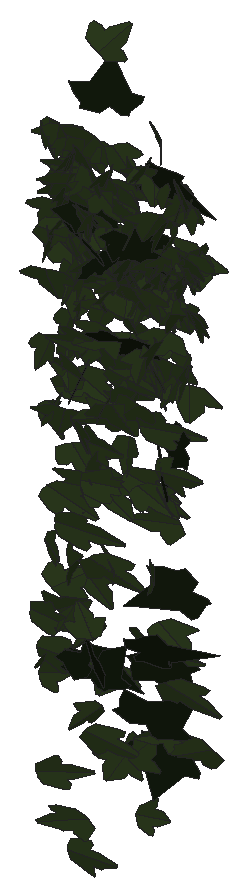
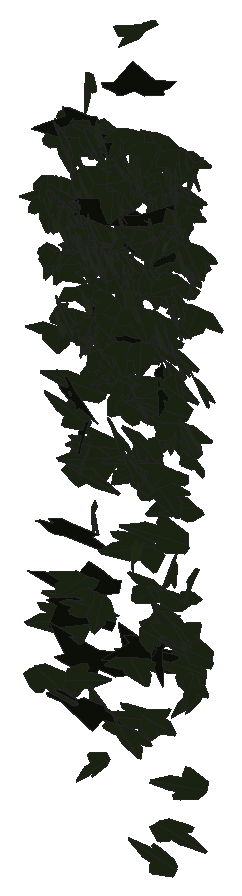
# SketchUp Ruby script. Lengths in millimetres.
U = 1.mm
M = Sketchup.active_model
def pt(a) = Geom::Point3d.new(a.map { |v| v * U })
def face(e, loops, mat)
  f = e.add_face(loops[0].map { |a| pt(a) })
  loops[1..].each { |l| e.add_face(l.map { |a| pt(a) }).erase! }
  f.material = f.back_material = mat if mat
  f
end
# faces: each face lists its corners as indices into pts; further lists are holes
def faces(e, pts, list, mat = nil) = list.each { |f| face(e, (f[0].is_a?(Array) ? f : [f]).map { |l| l.map { |i| pts[i] } }, mat) }
# xy, xz, yz: faces in a plane at the given z, y or x. An outline is a flat list of corners, or four numbers for a rectangle; further outlines are holes
def ring(l) = l.size == 4 ? [[l[0], l[1]], [l[2], l[1]], [l[2], l[3]], [l[0], l[3]]] : l.each_slice(2).to_a
def flat(e, list, mat, &to3) = list.each { |f| face(e, (f[0].is_a?(Array) ? f : [f]).map { |l| ring(l).map { |u, v| to3.(u, v) } }, mat) }
def xy(e, z, list, mat = nil) = flat(e, list, mat) { |x, y| [x, y, z] }
def xz(e, y, list, mat = nil) = flat(e, list, mat) { |x, z| [x, y, z] }
def yz(e, x, list, mat = nil) = flat(e, list, mat) { |y, z| [x, y, z] }
def lines(e, pts, list) = list.each { |a, b| e.add_line(pt(pts[a]), pt(pts[b])) }
# prism: a flat outline (further loops are holes) pulled along v
def prism(e, loops, v, mat = nil)
  f = face(e, loops, mat); d = Geom::Vector3d.new(v.map { |x| x * U })
  f.pushpull(f.normal.samedirection?(d) ? d.length : -d.length)
end
def box(e, o, s, mat = nil) = prism(e, [[o, [o[0] + s[0], o[1], o[2]], [o[0] + s[0], o[1] + s[1], o[2]], [o[0], o[1] + s[1], o[2]]]], [0, 0, s[2]], mat)
def at(x, y, z, deg = 0) = Geom::Transformation.translation(pt([x, y, z])) * Geom::Transformation.rotation(ORIGIN, Z_AXIS, deg.degrees)
def axes(o, x, y, z) = Geom::Transformation.new([*x, 0, *y, 0, *z, 0, *pt(o).to_a, 1])
def part(name) = M.definitions.add(name)
# library, detail: a bought-in or finely detailed component or shape, given as its bounding box
def library(name, o, s) = part(name).tap { |d| box(d.entities, o, s) }
def detail(e, o, s) = box(e.add_group.entities, o, s)
def put(e, d, t, mat = nil) = e.add_instance(d, t).tap { |i| i.material = mat if mat }
def group(e, t, mat = nil) = e.add_group.tap { |g| g.transformation = t; g.material = mat if mat }.entities
root = M.entities
M.materials.add("efeu1").color = [18, 25, 13]
M.materials.add("efeu2").color = [43, 57, 29]
c1 = part("ivyleaf_10")
p = [[0,12.8,-0.8],[-1.5,51.3,-10.9],[-4.9,51,-11.6],[-13.6,26.5,-7.3],[-13.2,15.9,-4.6],[-21.1,19.3,-7.2],
  [-29.5,16.3,-8.3],[-29.2,8.3,-6.2],[-19.7,-9.8,0.5],[-7.6,-13,4],[1,-12.2,5.8],[-0.4,51.1,-11.1],
  [-1.5,51.1,-10.9],[1,-12.4,5.9],[16.9,-12.4,3.5],[35.1,9.1,-5.1],[35,12.9,-6.1],[20.5,16.4,-4.9],
  [15.8,15,-3.8],[15.3,27.6,-7.1],[12.8,31.3,-7.8]]
faces(c1.entities,p,[[0,1,2,3,4,5,6,7,8,9,10],[11,12,0,13,14,15,16,17,18,19,20]],"efeu2")
c2 = part("ivyleaf_9")
p = [[39.1,54.8,31.7],[34.5,51.8,30.2],[-5.3,25.2,17.3],[-17.9,28.3,20.9],[-21.6,21.7,17],[-20.2,4.3,5.3],
  [-22.9,-0.3,2.5],[-17.1,-4,-0.6],[-2,-2.1,-1.2],[-0.7,-15.4,-10.1],[16.6,-22.3,-16.7],[21.1,-15.1,-12.5],
  [32.7,-10.7,-11],[46.1,-1.8,-6.6],[30.8,11.2,3.8]]
faces(c2.entities,p,[[0,1,2,3,4,5,6,7,8,9,10,11,12,13,14]],"efeu1")
put(root,c1,axes([1869.2,1029.3,798.4],[0.90738,-0.48267,0.05189],[0.05263,-0.04561,-0.67832],[0.92241,0.47741,-0.01234]))
put(root,c1,axes([1871.8,1032,897.3],[-1.24405,-0.13361,-0.11217],[0.20532,0.03226,-0.6671],[0.26092,-0.66243,-0.00987]))
put(root,c1,axes([1875.6,1030.7,519.9],[-0.37912,0.53611,0.3744],[-0.30349,0.33975,-0.57133],[-1.20694,-0.25383,0.02606]))
put(root,c1,axes([1874.4,1033.8,369],[-0.21212,-0.54646,-0.44472],[0.17012,0.43564,-0.55771],[1.33007,-0.14287,0.00041]))
put(root,c1,axes([1874.3,1024.3,1105.1],[-0.16268,0.70253,0.12456],[-0.12748,0.117,-0.70583],[-1.35191,-0.09557,0.05157]))
put(root,c1,axes([1879.6,1037.5,989.3],[1.27986,0.02095,-0.20491],[-0.38647,0.18461,-0.64756],[0.06565,0.67833,0.18256]))
put(root,c1,axes([1876.4,1025.5,342.8],[-0.0711,0.23931,0.73813],[-0.18187,0.73194,-0.24214],[-1.46555,-0.10244,-0.00576]))
put(root,c1,axes([1879.4,1022.1,952.3],[0.18952,-0.45863,-0.5924],[0.06095,0.59967,-0.45888],[1.42455,0.03536,0.09845]))
put(root,c1,axes([1861.4,1048.1,698.6],[0.73815,-0.23679,0.45324],[0.79308,-0.18337,-0.45238],[0.56409,0.56765,0.04293]))
put(root,c1,axes([1875.8,1027.5,702.7],[0.39878,-0.71333,0.09203],[0.04553,0.10271,0.74168],[-1.36811,-0.20451,0.05151]))
put(root,c1,axes([1857.3,1035.8,413.5],[0.02097,0.0114,0.70069],[1.31077,0.12931,-0.01293],[-0.24643,0.68875,-0.00917]))
put(root,c1,axes([1887.8,1035.7,973.4],[0.23825,-0.69334,0.05727],[0.03936,-0.05446,-0.70447],[1.32347,0.12643,0.01064]))
put(root,c1,axes([1900,1017.8,1106.3],[0.50659,-0.48712,-0.4683],[-0.4436,0.40624,-0.55505],[1.20709,0.35373,-0.00744]))
put(root,c1,axes([1890,1046,835.6],[0.77843,-0.48828,0.13906],[0.14957,-0.11552,-0.63681],[0.95459,0.41627,-0.01362]))
put(root,c1,axes([1897,1032,1032.3],[-0.51019,-0.65992,-0.06819],[0.04332,0.06435,-0.71228],[1.2619,-0.26902,-0.00312]))
put(root,c1,axes([1901.4,1025.6,716.5],[-1.11368,-0.33892,0.084],[-0.12948,-0.05012,-0.67616],[0.65181,-0.58903,0.00921]))
put(root,c1,axes([1893.6,1042.6,804.4],[0.2337,0.61212,-0.19031],[-0.1827,-0.17402,-0.62168],[-1.20623,0.14495,0.05729]))
put(root,c1,axes([1914.6,1035.5,145.8],[0.70854,0.0556,-0.56665],[-1.0806,-0.01434,-0.37444],[-0.08097,0.67785,0.03856]))
put(root,c1,axes([1900.4,1028.7,1110.1],[-0.96496,-0.51288,0.04323],[0.11399,-0.11907,-0.71008],[0.97292,-0.49474,0.12607]))
put(root,c1,axes([1899.9,1040.7,922.4],[0.81679,-0.52205,-0.12273],[-0.09683,0.11685,-0.67494],[1.01605,0.43081,0.03434]))
put(root,c1,axes([1883,1019.7,208],[-0.12187,-0.11847,0.71745],[0.66916,0.62539,0.13465],[-1.21141,0.35737,0.0022]))
put(root,c1,axes([1878.7,1024.3,966.6],[-0.35032,-0.14395,-0.67044],[1.20953,0.22489,-0.22277],[0.49012,-0.65787,0.07055]))
put(root,c1,axes([1902.7,1028.5,1030.1],[0.14499,-0.70911,-0.035],[0.02921,0.03684,-0.71293],[1.3509,0.07531,0.01917]))
put(root,c1,axes([1902.1,1042.7,812.7],[0.84625,-0.4996,-0.08924],[-0.08285,0.08067,-0.66848],[0.96233,0.44628,0.02093]))
put(root,c1,axes([1921.6,1019.6,778.5],[0.10379,-0.07883,-0.71109],[-0.96747,0.49756,-0.09414],[0.95815,0.51094,-0.01803]))
put(root,c1,axes([1902,1034.8,437.4],[0.87978,-0.51846,-0.03595],[-0.04796,0.0257,-0.69461],[0.98793,0.46294,-0.0017]))
put(root,c1,axes([1904.6,1038.2,892.7],[0.49545,-0.64141,-0.04392],[-0.02861,0.0413,-0.69222],[1.22326,0.26075,0.0016]))
put(root,c1,axes([1909.4,1024.3,1048.7],[-0.79443,-0.57764,0.05217],[-0.05687,-0.04278,-0.71267],[1.10237,-0.41849,0.00083]))
put(root,c1,axes([1911.8,1030.2,1057.9],[-1.34835,-0.08584,0.09967],[-0.18559,-0.0237,-0.71355],[0.16801,-0.71505,0.01169]))
put(root,c1,axes([1893,1037,432.7],[-1.03722,-0.17404,0.38096],[0.70107,0.09836,0.5719],[-0.37937,0.65762,0.01528]))
put(root,c1,axes([1887.5,1041.8,937.6],[0.87129,0.2454,0.46092],[0.75076,0.23911,-0.51911],[-0.65117,0.60404,0.01823]))
put(root,c1,axes([1923.8,1025.5,1002.4],[-0.81102,0.38818,0.4143],[-0.78257,0.14618,-0.55989],[-0.74506,-0.57608,0.1371]))
put(root,c1,axes([1914.5,1029.9,1004.8],[-1.23448,0.26015,0.1042],[-0.16954,0.05768,-0.69857],[-0.50569,-0.65441,-0.02015]))
put(root,c1,axes([1912.4,1022.8,1084.5],[0.37192,-0.65065,-0.2868],[-0.0069,0.29652,-0.67517],[1.35327,0.18033,0.07538]))
put(root,c1,axes([1918.7,1025.1,1092.9],[-0.98634,0.43433,0.25704],[-0.42293,0.13441,-0.67517],[-0.8624,-0.56266,0.03713]))
put(root,c1,axes([1893.6,1027.9,474.2],[0.72081,0.16976,-0.59681],[0.89097,0.38073,0.40538],[0.77507,-0.59554,0.08903]))
put(root,c1,axes([1913.9,1024.8,1080.8],[-0.01475,-0.69357,-0.19751],[0.05754,0.19703,-0.69308],[1.37127,-0.01573,0.02696]))
put(root,c1,axes([1883.2,1023.3,377.6],[-0.02616,0.02185,-0.77796],[1.4554,-0.14422,-0.01756],[-0.27527,-0.7646,-0.01892]))
put(root,c1,axes([1907.8,1044.4,879.5],[1.24386,-0.13508,0.0773],[0.13939,-0.0275,-0.66727],[0.26135,0.65754,-0.01202]))
put(root,c1,axes([1920.8,1030.1,912.8],[0.60241,-0.53759,-0.39212],[-0.23928,0.37809,-0.61983],[1.24358,0.33316,0.07069]))
put(root,c1,axes([1913.7,1050.7,867.1],[0.24232,-0.63004,0.19354],[0.19168,-0.1762,-0.63986],[1.23966,0.1504,0.0611]))
put(root,c1,axes([1911.6,1033.9,959.6],[-0.23603,0.68197,0.07052],[0.00464,0.0721,-0.69298],[-1.30483,-0.12311,-0.01522]))
put(root,c1,axes([1897.8,1035.7,746.9],[-0.30774,-0.16716,0.65401],[0.79369,0.50409,0.23194],[-1.01024,0.44696,-0.017]))
put(root,c1,axes([1917.7,1017.1,514.2],[0.15685,-0.2596,-0.77329],[0.08281,0.77752,-0.25638],[1.55023,-0.01526,0.09194]))
put(root,c1,axes([1922.6,1027.9,977.8],[0.15997,0.2002,-0.74136],[-0.17654,0.74297,0.19012],[1.45079,0.06834,0.10488]))
put(root,c1,axes([1937.5,1023.1,825.4],[0.52602,0.02308,-0.64568],[-1.17735,0.21208,-0.25722],[0.35478,0.66956,0.10373]))
put(root,c1,axes([1910.1,1027.2,1049.3],[-1.13091,-0.32991,-0.26224],[0.57378,-0.01601,-0.66299],[0.56046,-0.64931,0.14959]))
put(root,c1,axes([1932.3,1032.3,627.5],[-1.07139,-0.21896,0.34265],[-0.58476,-0.15427,-0.60337],[0.50694,-0.64071,0.02818]))
put(root,c1,axes([1897.3,1018.7,605.3],[0.64467,0.28691,0.5898],[0.86938,0.37315,-0.44386],[-0.89575,0.56865,-0.00632]))
put(root,c1,axes([1925.6,1033.7,973.2],[-0.89693,-0.50798,0.10975],[-0.02806,-0.13503,-0.68828],[0.98869,-0.46466,0.08003]))
put(root,c1,axes([1916.8,1028.6,706.1],[-0.77464,0.51378,-0.15067],[0.16318,-0.12427,-0.65539],[-1.00585,-0.41584,0.00971]))
put(root,c1,axes([1919,1025.3,1063],[1.26036,-0.30568,0.00153],[0.01934,0.01837,-0.72908],[0.58145,0.66198,0.02094]))
put(root,c2,axes([1932.9,1014.6,774.3],[-0.24355,0.15475,-0.77354],[-1.03911,0.54826,0.2],[1.08368,0.56049,0.01793]))
put(root,c1,axes([1909.5,1039.3,659],[1.01715,0.34047,0.27122],[0.42607,0.15334,-0.63363],[-0.7105,0.57938,0.00831]))
put(root,c1,axes([1919.6,1037.7,989.8],[0.03741,-0.59176,-0.37503],[0.34064,0.36697,-0.56966],[1.28912,-0.0798,0.16141]))
put(root,c1,axes([1922.7,1035.2,964.5],[-1.30315,-0.08826,-0.11103],[0.2088,0.01732,-0.69037],[0.17107,-0.69344,-0.00311]))
put(root,c1,axes([1930.1,1047.7,299.9],[-0.16769,-0.42013,0.50884],[-0.11506,-0.50606,-0.4283],[1.25058,-0.1029,0.02882]))
put(root,c1,axes([1918.7,1022.7,1038.4],[-1.07164,-0.26725,-0.35085],[0.58386,0.17146,-0.62295],[0.60307,-0.6409,-0.02035]))
put(root,c2,axes([1904.6,1035.1,978.8],[0.71859,-0.64527,0.24174],[0.23485,-0.20787,-0.74761],[1.29022,0.39722,0.00145]))
put(root,c1,axes([1933.7,1043.5,928.2],[-0.33889,-0.66496,0.00959],[0.01809,-0.01247,-0.68827],[1.26555,-0.17789,0.01241]))
put(root,c1,axes([1955.1,1032.3,991.7],[0.51592,-0.01403,-0.65537],[-1.19211,0.20358,-0.26344],[0.36788,0.67937,0.06541]))
put(root,c2,axes([1946.9,1032.4,997.9],[-1.2663,-0.37347,0.21608],[0.40405,0.06237,0.76151],[-0.71491,0.69677,0.04765]))
put(root,c1,axes([1939.3,1042.1,420.2],[-0.05524,-0.42579,0.51823],[-0.0381,-0.51794,-0.42667],[1.27595,-0.0339,0.0097]))
put(root,c1,axes([1908.4,1027.1,557.9],[0.03304,-0.04195,0.81892],[1.4007,0.36199,0.00294],[-0.68817,0.73478,0.0453]))
put(root,c1,axes([1940.5,1023.1,426],[0.43203,0.6509,0.02879],[-0.01824,-0.02714,0.68935],[1.23987,-0.22721,0.00011]))
put(root,c1,axes([1913.6,1039.7,97.5],[0.22404,-0.05782,-0.69253],[1.16936,-0.31951,0.13112],[-0.61795,-0.62559,-0.00296]))
put(root,c1,axes([1937.7,1025.6,1065.2],[1.05261,-0.42964,-0.20857],[0.02297,0.33159,-0.65106],[0.90865,0.48933,0.25806]))
put(root,c1,axes([1945,1019.4,1115.2],[1.23119,-0.19465,-0.31456],[-0.4179,0.30792,-0.6421],[0.56658,0.65009,0.20995]))
put(root,c1,axes([1938.4,1026.4,1103.8],[-1.23328,-0.29707,-0.16107],[0.33988,-0.00533,-0.70864],[0.54599,-0.6677,0.07732]))
put(root,c1,axes([1920,1044.8,487.7],[1.09364,0.06195,0.46136],[0.86422,0.08666,-0.57722],[-0.19492,0.73181,0.02929]))
put(root,c2,axes([1955,1016.1,398.3],[0.444,0.0027,-0.75716],[-1.39505,0.19936,-0.22514],[0.36113,0.76679,0.0612]))
put(root,c1,axes([1946.9,1022.6,652.1],[-0.17277,0.27104,0.60208],[-0.40048,0.56418,-0.28571],[-1.19112,-0.229,0.00873]))
put(root,c1,axes([1942.1,1027.4,1003.2],[0.12581,-0.70793,-0.03914],[0.20415,0.04884,-0.70226],[1.33385,0.0593,0.11118]))
put(root,c1,axes([1924.9,1031.1,772.1],[0.7651,0.41206,0.50055],[0.69141,0.34465,-0.57549],[-1.02201,0.54164,-0.01461]))
put(root,c1,axes([1952.4,1045.3,872.3],[-1.01897,-0.36098,0.13926],[-0.14907,-0.13172,-0.64255],[0.72112,-0.5373,0.06395]))
put(root,c1,axes([1963.1,1037.1,918.4],[0.85012,0.24064,-0.45675],[-0.97884,0.15486,-0.42138],[-0.08551,0.61981,0.28262]))
put(root,c1,axes([1970.6,1035.5,731.3],[-0.56478,-0.17989,0.61317],[-0.92096,-0.37828,-0.34517],[0.79429,-0.56652,0.03577]))
put(root,c1,axes([1951.6,1039.9,820.8],[-0.44554,-0.60072,-0.16652],[0.14091,0.14982,-0.64457],[1.17801,-0.24513,0.01412]))
put(root,c1,axes([1965.2,1022.6,848.5],[1.04645,-0.14115,-0.43031],[-0.77415,0.14363,-0.56686],[0.37891,0.68327,0.03027]))
put(root,c1,axes([1935.1,1040.4,676.5],[-0.50971,0.06887,0.65345],[1.20446,-0.16273,0.27653],[0.3363,0.6872,0]))
put(root,c2,axes([1935.3,1023.7,389.8],[0.03833,-0.20481,-0.73651],[0.68448,0.65268,-0.17166],[1.28385,-0.34186,0.11351]))
put(root,c1,axes([1959.3,1038.2,751.4],[0.45401,-0.67456,0.04375],[0.03265,-0.04034,-0.71549],[1.2861,0.23915,0.00272]))
put(root,c2,axes([1948.8,1022,365.4],[-0.8567,0.16075,0.59626],[1.04883,-0.22842,0.47762],[0.53041,0.71132,0.01862]))
put(root,c1,axes([1941.4,1045.8,634.2],[0.50849,-0.29727,-0.61621],[0.75646,-0.471,0.39955],[-1.05982,-0.47881,-0.01046]))
put(root,c1,axes([1963.9,1042.1,898.5],[-0.07625,-0.66463,-0.04561],[0.01867,0.0451,-0.6658],[1.26776,-0.04064,0.00706]))
put(root,c1,axes([1962.7,1042.5,369.6],[1.11396,0.32787,-0.18661],[-0.325,-0.07689,-0.6707],[-0.64022,0.60951,0.01577]))
put(root,c2,axes([1964.5,1010,945.4],[-0.69895,0.64319,-0.28504],[-0.2727,0.24642,0.74065],[1.31088,0.39421,0.0021]))
put(root,c1,axes([1945.9,1037.8,979.3],[0.61143,0.31857,0.53996],[0.65471,0.41766,-0.45109],[-0.99751,0.4694,0.03491]))
put(root,c1,axes([1965.2,1033.5,987.2],[-0.28251,0.67141,-0.15233],[-0.09529,-0.16594,-0.68263],[-1.30684,-0.13305,0.08271]))
put(root,c1,axes([1971.9,1023,1079.4],[-0.10492,-0.67514,-0.28163],[0.00385,0.28228,-0.67711],[1.39223,-0.05166,-0.01935]))
put(root,c1,axes([1972.5,1039.1,813.2],[-1.09428,-0.34902,-0.06739],[0.10707,0.03718,-0.6726],[0.66799,-0.57771,-0.00258]))
put(root,c1,axes([1960.1,1043.2,518],[-0.39992,0.10814,0.66432],[0.80799,-0.51874,0.21873],[0.99401,0.46517,0.08948]))
put(root,c1,axes([1976.3,1044,932.3],[-0.71874,-0.57098,0.05906],[0.04805,-0.08715,-0.6811],[1.09144,-0.37217,0.06888]))
put(root,c2,axes([1975.9,1021.3,1177.3],[-1.13627,-0.25849,0.507],[0.89507,0.18966,0.65051],[-0.60987,0.75995,0.0101]))
put(root,c1,axes([1966.4,1025.8,1038.1],[0.82026,0.45239,0.33799],[0.08856,0.39528,-0.58841],[-1.07109,0.37913,0.21019]))
put(root,c1,axes([1981.4,1027.2,820.9],[-1.23012,-0.13021,0.09156],[-0.17089,-0.01792,-0.65933],[0.25014,-0.65255,-0.00016]))
put(root,c1,axes([1976.7,1043.7,913.1],[-0.59365,-0.60076,-0.06235],[0.12042,0.03728,-0.6758],[1.14319,-0.3159,0.03881]))
put(root,c1,axes([1979.5,1032,929.3],[-0.5486,0.57807,0.22661],[-0.23821,0.19062,-0.64545],[-1.15745,-0.31322,0.02543]))
put(root,c1,axes([1954.5,1025.2,281.7],[-0.5241,-0.01575,-0.69148],[1.31617,-0.01937,-0.27497],[-0.02316,-0.74405,0.0218]))
put(root,c1,axes([1958.9,1013.1,641.9],[0.09116,0.03506,0.74705],[0.83284,0.60574,-0.05648],[-1.15426,0.43983,0.01824]))
put(root,c1,axes([2002.4,1024.3,1038.4],[0.34132,0.00919,0.70771],[-1.32016,0.1474,0.17386],[-0.26775,-0.71505,0.04493]))
put(root,c1,axes([1971.8,1014.3,1260.1],[0.62985,0.25071,-0.71224],[0.56946,0.67044,0.37503],[1.31942,-0.40904,0.17814]))
put(root,c1,axes([1961.5,1022.7,527],[-0.94004,-0.07334,-0.62422],[1.18806,0.03515,-0.49807],[0.13921,-0.79522,0.03556]))
put(root,c1,axes([1984.3,1032.4,947.6],[-0.67759,0.5905,0.14518],[-0.19554,0.1074,-0.68879],[-1.14067,-0.36919,0.03183]))
put(root,c1,axes([1965.7,1018.6,634.7],[0.83196,0.41463,0.44634],[0.64025,0.29372,-0.60232],[-0.96665,0.5514,-0.01479]))
put(root,c1,axes([1985.6,1039.6,942.9],[0.76677,-0.5514,-0.11074],[-0.03267,0.1241,-0.68038],[1.06988,0.39897,0.05859]))
put(root,c1,axes([1987.6,1027.8,1054.6],[-1.12329,0.40233,-0.00681],[-0.13021,-0.11225,-0.70213],[-0.75467,-0.57948,0.13128]))
put(root,c1,axes([1986.6,1031.5,258.6],[1.27446,-0.14152,-0.14354],[-0.26775,0.02853,-0.68443],[0.27475,0.68426,-0.00115]))
put(root,c1,axes([1981.1,1027.4,747.1],[-1.20834,-0.34234,-0.28304],[0.47236,0.13607,-0.72131],[0.70111,-0.68169,-0.00184]))
put(root,c1,axes([1979.4,1039.6,923],[1.29431,-0.01999,0.0766],[0.15058,0.14965,-0.66341],[0.00501,0.66781,0.15096]))
put(root,c1,axes([2005.9,1026,1086.4],[-0.39237,0.11741,0.68981],[-1.08644,0.38766,-0.23659],[-0.77016,-0.60668,-0.01768]))
put(root,c1,axes([1982.3,1028.5,1061],[-1.29777,0.00203,-0.23138],[0.43876,-0.05572,-0.6799],[-0.03773,-0.71792,0.05211]))
put(root,c2,axes([1993.3,1020,853],[0.98689,0.41964,-0.39361],[-0.60776,-0.23085,-0.66682],[-0.91085,0.60871,0.01846]))
put(root,c1,axes([1981.9,1025.8,1110.1],[-0.81771,-0.53371,-0.25998],[0.58635,0.07387,-0.6608],[0.96579,-0.49672,0.18107]))
put(root,c1,axes([1993.5,1041.3,939.8],[0.17215,-0.68841,-0.00253],[-0.02961,0.00051,-0.69416],[1.30986,0.09049,-0.01536]))
put(root,c1,axes([1982,1047.5,690.6],[0.92764,-0.40839,0.33505],[0.46982,-0.22695,-0.63574],[0.88881,0.54619,-0.01364]))
put(root,c1,axes([1992.6,1042.3,941.2],[-1.11505,-0.32862,-0.12945],[0.27672,0.00409,-0.66847],[0.61261,-0.6,0.06634]))
put(root,c1,axes([1999.8,1029.5,1007],[0.42642,-0.5516,-0.38764],[-0.22824,0.36937,-0.59491],[1.26265,0.25305,0.02338]))
put(root,c1,axes([2009.6,1028.6,760.7],[-1.16475,-0.05726,0.34253],[-0.64583,-0.04897,-0.61449],[0.14053,-0.69962,0.01498]))
put(root,c1,axes([2000.2,1027,961.1],[0.10598,-0.70385,0.02087],[-0.0027,-0.02105,-0.70604],[1.34015,0.05562,-0.00307]))
put(root,c1,axes([1992.6,1032.3,890],[1.26355,0.24782,-0.06113],[0.10675,0.02453,0.70865],[0.47392,-0.66627,0.00335]))
put(root,c1,axes([2005.4,1035.2,1023.3],[-1.26552,0.20978,0.13214],[-0.25343,0.01687,-0.69686],[-0.39803,-0.67774,0.02356]))
put(root,c1,axes([2001.4,1044.2,940.4],[0.39991,-0.64611,0.10223],[0.02853,-0.10259,-0.6792],[1.24464,0.20995,-0.01727]))
put(root,c1,axes([1992.3,1032.7,780.8],[-0.50678,-0.36141,-0.54956],[0.6369,0.43598,-0.44886],[1.0777,-0.4276,0.00684]))
put(root,c1,axes([2006.1,1032.6,941.7],[-0.50964,0.46878,0.42568],[-0.38882,0.3735,-0.53984],[-1.14068,-0.33676,-0.00617]))
put(root,c1,axes([2006.4,1032.8,909.7],[0.58348,-0.61002,-0.07226],[-0.07599,0.0608,-0.68268],[1.16664,0.30905,-0.00833]))
put(root,c1,axes([2010.3,1043.9,790.8],[-0.62956,-0.59425,0.12127],[-0.08388,-0.11421,-0.67991],[1.15124,-0.33329,0.01678]))
put(root,c1,axes([1994.4,1039,843.2],[1.24631,0.18999,0.14129],[0.26014,0.03595,-0.68184],[-0.36794,0.66895,-0.00349]))
put(root,c1,axes([1984.8,1031.4,796.9],[-0.50888,-0.01656,-0.65176],[1.23311,-0.08527,-0.26363],[-0.13831,-0.6993,0.04759]))
put(root,c1,axes([2012.6,1037.9,941.4],[-0.33098,-0.6615,0.03756],[0.02853,-0.04275,-0.6835],[1.26066,-0.17271,0.02533]))
put(root,c1,axes([2005.4,1036.6,868.8],[-1.03339,0.35357,-0.15906],[0.23506,-0.10172,-0.64772],[-0.69943,-0.55658,0.01734]))
put(root,c1,axes([2010.5,1044,921.5],[0.56074,-0.61908,-0.05153],[0.02009,-0.05203,0.6855],[-1.18214,-0.29454,-0.01279]))
put(root,c1,axes([2023.2,1036.5,432.2],[-1.24818,0.39283,0.12554],[-0.20916,0.06083,-0.76447],[-0.75651,-0.66496,0.00423]))
put(root,c1,axes([2018.3,1034.7,911],[0.82907,-0.50722,0.1045],[0.1208,-0.08323,-0.66858],[0.97818,0.44018,-0.006]))
put(root,c1,axes([2031.7,1036.2,816.2],[0.82737,-0.32539,-0.48302],[-0.58096,0.38602,-0.53477],[0.94397,0.52277,0.09424]))
put(root,c1,axes([2021.2,1032.2,834.4],[-0.33941,-0.63529,0.24202],[0.23343,-0.27617,-0.63455],[1.27262,-0.11878,0.18094]))
put(root,c1,axes([2025.3,1047.4,938.7],[0.21862,-0.66534,0.07138],[-0.00579,-0.07295,-0.67501],[1.27353,0.11389,-0.01532]))
put(root,c1,axes([2008,1033.7,269.9],[1.09189,-0.41831,-0.27874],[0.46401,-0.13834,0.7094],[-0.83663,-0.62266,0.02966]))
put(root,c1,axes([2030.5,1041.8,941.3],[1.17711,-0.11408,-0.25369],[-0.44229,0.12799,-0.62411],[0.29094,0.65613,0.07764]))
put(root,c1,axes([2028.4,1024.8,1103.6],[0.10808,-0.72834,-0.05716],[0.01238,0.05783,-0.73047],[1.39038,0.0561,0.01095]))
put(root,c2,axes([2007.1,1026.8,998.2],[-0.18019,-0.33999,-0.74396],[0.56861,0.68281,-0.35007],[1.4492,-0.31018,0.04485]))
put(root,c1,axes([2020.2,1022.8,925.3],[-1.2345,0.03739,-0.22953],[0.43738,-0.00107,-0.64962],[-0.06777,-0.68806,-0.01146]))
put(root,c1,axes([2027.3,1047.9,933.1],[0.72091,0.52939,-0.18848],[-0.23355,-0.14389,-0.65077],[-1.04367,0.39787,0.01543]))
put(root,c1,axes([2038.4,1030.7,822.2],[-0.7005,0.50743,0.34833],[-0.436,0.26376,-0.62629],[-1.08723,-0.43271,0.02672]))
put(root,c1,axes([2028.5,1024.9,195.2],[-0.04994,0.29922,0.63077],[-0.03315,0.63073,-0.29993],[-1.32828,-0.02699,-0.01623]))
put(root,c1,axes([2030.7,1039.5,972.9],[0.71409,-0.58849,0.03217],[0.11149,-0.00071,-0.69621],[1.11614,0.37658,0.04896]))
put(root,c1,axes([2037.1,1035.2,965.1],[-1.30479,0.0927,0.02838],[-0.06824,-0.05418,-0.68934],[-0.17143,-0.68402,0.05844]))
put(root,c1,axes([2041.9,1030.5,1035.2],[-0.72491,-0.58178,0.17553],[-0.13555,-0.163,-0.69478],[1.14857,-0.38642,0.02879]))
put(root,c1,axes([2010.1,1032,657.8],[0.45349,0.13975,0.65069],[1.1012,0.298,-0.27588],[-0.62586,0.62559,-0.01394]))
put(root,c1,axes([2030.2,1043.1,837.6],[0.14922,0.66805,0.02246],[0.0087,0.02208,-0.67263],[-1.27213,0.07851,-0.00197]))
put(root,c1,axes([2056.6,1037.4,610.2],[0.52707,-0.06751,-0.63438],[-1.1966,0.08832,-0.28387],[0.20577,0.68653,-0.02586]))
put(root,c1,axes([2039.7,1037,969.2],[-0.63311,-0.61988,-0.05908],[0.06719,0.0481,-0.70345],[1.18319,-0.33442,0.00833]))
put(root,c1,axes([2043.9,1026.7,1099.7],[-1.19282,-0.36102,0.03365],[-0.05459,-0.01763,-0.72329],[0.68792,-0.6274,0.00096]))
put(root,c1,axes([2040.7,1046,948],[0.18417,-0.62053,0.2652],[0.05908,-0.26354,-0.62796],[1.28297,0.10121,-0.00915]))
put(root,c1,axes([2045.7,1035.1,648.7],[-0.70762,0.5281,0.30284],[-0.34392,0.24311,-0.64581],[-1.10638,-0.41333,0.00707]))
put(root,c1,axes([2049.3,1027,1089.4],[0.95716,-0.56422,-0.30564],[-0.41439,0.21525,-0.75562],[1.14881,0.54774,-0.0179]))
put(root,c1,axes([2021.9,1037.6,640],[-0.71814,-0.02111,-0.58524],[1.11366,0.01436,-0.37779],[0.04474,-0.69619,0.00996]))
put(root,c1,axes([2044.9,1028.5,859.7],[0.14449,-0.70488,0.09799],[0.03861,-0.09636,-0.70889],[1.35388,0.07798,0.00976]))
put(root,c1,axes([2033.2,1040.8,959.9],[-0.93419,0.27056,-0.40221],[0.51,-0.32555,-0.54601],[-0.76878,-0.54473,0.12654]))
put(root,c1,axes([2050.5,1011.1,539.8],[0.00001,-0.08958,-0.67894],[-0.19439,0.67135,-0.08858],[1.28879,0.10126,-0.01336]))
put(root,c1,axes([2056.8,1044.2,313.6],[0.09857,0.09369,-0.70529],[-0.87743,-0.5342,-0.10482],[-1.03137,0.46342,0.02177]))
put(root,c1,axes([2050.7,1035.7,868.9],[0.8573,0.37582,-0.33486],[-0.59907,-0.14034,-0.58094],[-0.74757,0.54345,0.08154]))
put(root,c1,axes([2043.4,1027.2,806.5],[-0.49131,0.63815,0.07496],[-0.0555,0.06906,-0.68838],[-1.22161,-0.25979,0.00113]))
put(root,c2,axes([2052.5,1037.5,654.7],[-0.03045,-0.41579,0.66314],[0.2541,0.6521,0.41209],[-1.46782,0.12151,0.05758]))
put(root,c1,axes([2030,1026.2,647.9],[0.66816,0.35443,0.47626],[0.59941,0.35783,-0.49845],[-0.95776,0.4712,0.02029]))
put(root,c1,axes([2041.8,1025.9,1097],[1.16113,0.38909,-0.0028],[-0.01496,0.00711,-0.72353],[-0.74038,0.61006,0.01022]))
put(root,c1,axes([2051.1,1043.7,943.2],[0.65645,-0.55655,-0.19979],[-0.13958,0.18925,-0.65379],[1.11672,0.35081,0.03573]))
put(root,c2,axes([2050.3,1044.3,284.9],[-1.36287,-0.28278,-0.3521],[0.62764,0.1235,-0.76988],[0.58717,-0.78836,0.00569]))
put(root,c1,axes([2031.5,1043,910.8],[0.43062,-0.32432,0.5422],[1.00698,-0.21748,-0.35088],[0.65715,0.54578,0.18237]))
put(root,c1,axes([2052.6,1029.1,1027.8],[0.29207,-0.69055,0.08481],[0.06601,-0.07915,-0.7072],[1.32249,0.15646,0.01657]))
put(root,c1,axes([2042.4,1031.5,925.2],[-1.12804,-0.09398,-0.31926],[0.63316,-0.18537,-0.56305],[-0.01754,-0.6472,0.20763]))
put(root,c1,axes([2062,1038.2,829.1],[-1.2423,-0.09316,0.14039],[-0.25063,-0.06832,-0.65761],[0.20004,-0.66416,0.04796]))
put(root,c2,axes([2035.8,1023,329],[-0.67939,0.12119,0.75407],[1.35749,-0.24468,0.37698],[0.51967,0.79761,0.00107]))
put(root,c2,axes([2079.1,1035.4,725.3],[-0.43127,0.0833,-0.7197],[-1.34614,0.1379,0.23866],[0.29867,0.74182,0.03645]))
put(root,c1,axes([2059.1,1040,978.9],[-0.48474,-0.64705,0.0378],[0.02238,-0.04522,-0.69483],[1.23336,-0.25349,0.02747]))
put(root,c1,axes([2057.7,1014.5,1157.8],[0.59402,-0.4556,-0.5088],[-0.03513,0.55359,-0.50702],[1.29935,0.22325,0.2189]))
put(root,c1,axes([2056.5,1041.2,964],[0.39479,-0.65308,0.08528],[0.07619,-0.07674,-0.68508],[1.25119,0.21074,0.01481]))
put(root,c1,axes([2032.5,1035.9,734.1],[-0.26116,-0.08647,0.76358],[1.23158,0.40535,0.16219],[-0.78882,0.6615,0.00042]))
put(root,c2,axes([2045.2,1033,415.1],[-0.4162,-0.36976,-0.64994],[0.62624,0.56049,-0.42959],[1.27794,-0.39509,-0.00116]))
put(root,c1,axes([2038.2,1034.3,420.9],[-0.12236,-0.11668,0.69634],[1.1037,0.39011,0.11892],[-0.76648,0.58037,0.06007]))
put(root,c2,axes([2085.2,1040.9,522.9],[-1.47744,-0.06747,0.23343],[-0.43935,-0.03911,-0.77901],[0.14433,-0.80968,0.01818]))
put(root,c1,axes([2049.5,1039.4,457.2],[0.70957,0.50135,0.35477],[0.41004,0.28188,-0.62477],[-1.09462,0.43059,-0.00406]))
put(root,c2,axes([2034.5,1015.9,431.5],[0.55363,0.02408,0.75124],[1.41895,0.0929,-0.29167],[-0.18139,0.80022,0.01125]))
put(root,c1,axes([2064.5,1032.1,809.4],[0.73804,-0.55151,0.00364],[0.00437,-0.00284,-0.6742],[1.04965,0.3878,0.00025]))
put(root,c1,axes([2082.1,1046.9,896.3],[-1.0449,0.02235,-0.40135],[-0.76292,0.02003,0.54947],[0.05684,0.67978,-0.00299]))
put(root,c1,axes([2069.4,1028,1021.4],[0.24862,-0.67134,-0.19616],[-0.05897,0.1938,-0.68391],[1.32982,0.13411,0.00635]))
put(root,c2,axes([2037.7,1024.5,1098.5],[0.0477,-0.00634,-0.81179],[1.28552,0.4507,0.01734],[0.85709,-0.67564,0.01918]))
put(root,c1,axes([2075,1030.9,983],[-1.02157,0.44477,0.03747],[-0.18236,-0.05758,-0.68909],[-0.82968,-0.53498,0.10532]))
put(root,c1,axes([2072.4,1047.1,841.2],[0.77238,-0.54322,0.02309],[0.0233,-0.01968,-0.67808],[1.03453,0.40601,-0.00197]))
put(root,c1,axes([2081.9,1028.2,1071],[-1.30377,0.16311,0.18269],[-0.36737,-0.02557,-0.70096],[-0.28688,-0.70852,0.06735]))
put(root,c1,axes([2072.8,1039.6,980.7],[0.73123,-0.57202,-0.11484],[0.03907,0.15067,-0.68183],[1.1097,0.37162,0.09968]))
put(root,c1,axes([2077.9,1039.8,975.4],[1.03915,-0.39262,-0.12601],[-0.20955,0.06268,-0.67238],[0.75628,0.55684,-0.01316]))
put(root,c1,axes([2073,1039.9,909.8],[-0.48269,-0.58125,-0.24503],[0.33022,0.18962,-0.62941],[1.1542,-0.29733,0.07761]))
put(root,c1,axes([2096.7,1041.6,996.8],[-0.94171,0.16819,0.44755],[-0.90761,-0.21967,-0.44469],[0.06505,-0.62998,0.27454]))
put(root,c1,axes([2074.8,1023.7,916.3],[-0.11778,-0.32946,-0.66162],[0.33762,0.63791,-0.33424],[1.36556,-0.18613,0.02557]))
put(root,c1,axes([2079.4,1028.1,1072.1],[0.50774,-0.66212,-0.10822],[0.09055,0.13484,-0.7077],[1.27365,0.25437,0.09346]))
put(root,c1,axes([2081,1037.7,977.2],[-0.89727,0.51453,0.03959],[-0.06821,0.02085,-0.69775],[-0.97977,-0.47266,0.01232]))
put(root,c1,axes([2056,1033.7,682.7],[0.36622,-0.08872,-0.67192],[1.11198,-0.33226,0.21119],[-0.6537,-0.6149,-0.01717]))
put(root,c1,axes([2104.2,1046.3,304.2],[-0.89631,-0.11357,0.54585],[-0.96616,-0.20807,-0.48128],[0.43871,-0.69025,0.05527]))
put(root,c1,axes([2079.2,1043.7,826.5],[0.31221,-0.57953,0.34818],[0.32207,-0.31168,-0.59851],[1.24576,0.22582,0.06747]))
put(root,c1,axes([2086.5,1035.1,965],[-0.02023,-0.70751,-0.00159],[0.01494,0.00147,-0.70754],[1.34645,-0.01064,0.00783]))
put(root,c1,axes([2091.2,1022.6,997.3],[-1.16832,0.27502,0.1835],[-0.3234,0.06952,-0.67263],[-0.53976,-0.63693,0.00582]))
put(root,c1,axes([2096,1019.6,1072.5],[0.95085,-0.36196,-0.42016],[-0.55388,0.31027,-0.61334],[0.89845,0.57435,0.06655]))
put(root,c1,axes([2090.2,1036.8,983.8],[-0.32584,0.65872,0.16593],[-0.35235,0.1194,-0.665],[-1.2439,-0.20637,0.1449]))
put(root,c1,axes([2085.4,1020.6,1095.6],[-0.69558,0.631,-0.02428],[-0.01898,-0.03381,-0.72875],[-1.20166,-0.36472,0.02556]))
put(root,c1,axes([2091,1029.7,1081.8],[0.6544,-0.61946,-0.14752],[-0.09337,0.14138,-0.70804],[1.20832,0.34641,0.02518]))
put(root,c1,axes([2094.2,1025.1,1001.4],[-1.30159,-0.15676,0.04606],[-0.04862,-0.09317,-0.69647],[0.30713,-0.67908,0.08493]))
put(root,c1,axes([2092,1041.1,909.7],[-0.88963,0.48932,0.07753],[-0.1061,0.05397,-0.6767],[-0.9369,-0.47074,0.00301]))
put(root,c1,axes([2085.3,1040.2,801.7],[1.21098,0.29088,0.02502],[0.03466,0.02033,-0.69954],[-0.55456,0.63645,0.01091]))
put(root,c1,axes([2074,1030,387.5],[-0.92083,-0.02471,-0.61449],[1.16857,0.02478,-0.48445],[0.06615,-0.78171,0.00407]))
put(root,c1,axes([2097.7,1040.1,979.2],[-0.84976,-0.52236,-0.09133],[0.09753,0.07633,-0.6871],[1.00451,-0.4493,-0.01055]))
put(root,c1,axes([2100.5,1038.5,1004.3],[-0.17445,-0.68778,-0.07675],[0.17636,0.06452,-0.6889],[1.30525,-0.10064,0.08283]))
put(root,c1,axes([2097.9,1039.1,990.6],[0.87925,0.50867,0.01464],[-0.00391,0.02164,-0.68696],[-0.96849,0.46171,0.01607]))
